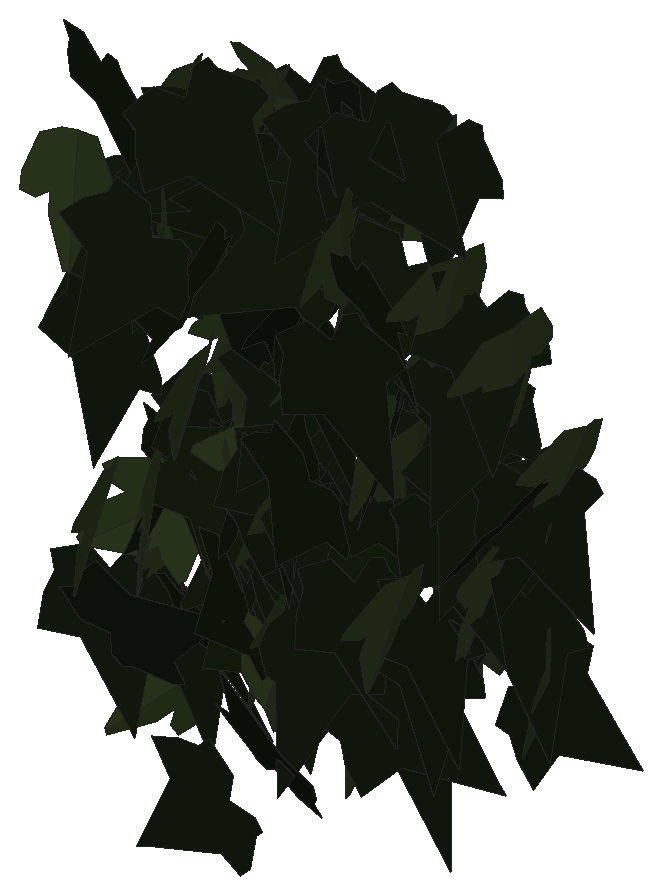
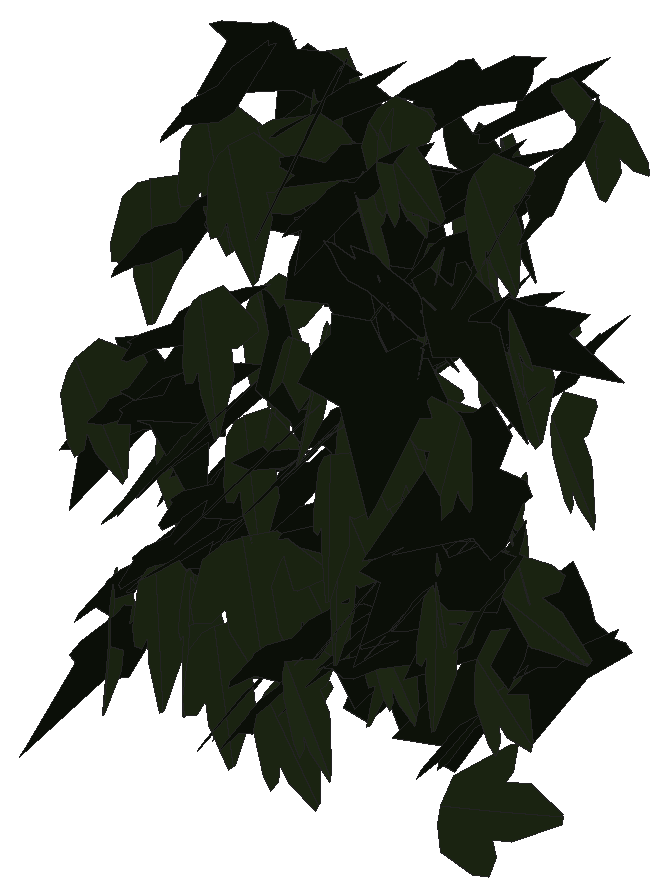
# SketchUp Ruby script. Lengths in inches.
U = 1.inch
M = Sketchup.active_model
def pt(a) = Geom::Point3d.new(a.map { |v| v * U })
def face(e, loops, mat)
  f = e.add_face(loops[0].map { |a| pt(a) })
  loops[1..].each { |l| e.add_face(l.map { |a| pt(a) }).erase! }
  f.material = f.back_material = mat if mat
  f
end
# faces: each face lists its corners as indices into pts; further lists are holes
def faces(e, pts, list, mat = nil) = list.each { |f| face(e, (f[0].is_a?(Array) ? f : [f]).map { |l| l.map { |i| pts[i] } }, mat) }
# xy, xz, yz: faces in a plane at the given z, y or x. An outline is a flat list of corners, or four numbers for a rectangle; further outlines are holes
def ring(l) = l.size == 4 ? [[l[0], l[1]], [l[2], l[1]], [l[2], l[3]], [l[0], l[3]]] : l.each_slice(2).to_a
def flat(e, list, mat, &to3) = list.each { |f| face(e, (f[0].is_a?(Array) ? f : [f]).map { |l| ring(l).map { |u, v| to3.(u, v) } }, mat) }
def xy(e, z, list, mat = nil) = flat(e, list, mat) { |x, y| [x, y, z] }
def xz(e, y, list, mat = nil) = flat(e, list, mat) { |x, z| [x, y, z] }
def yz(e, x, list, mat = nil) = flat(e, list, mat) { |y, z| [x, y, z] }
def lines(e, pts, list) = list.each { |a, b| e.add_line(pt(pts[a]), pt(pts[b])) }
# prism: a flat outline (further loops are holes) pulled along v
def prism(e, loops, v, mat = nil)
  f = face(e, loops, mat); d = Geom::Vector3d.new(v.map { |x| x * U })
  f.pushpull(f.normal.samedirection?(d) ? d.length : -d.length)
end
def box(e, o, s, mat = nil) = prism(e, [[o, [o[0] + s[0], o[1], o[2]], [o[0] + s[0], o[1] + s[1], o[2]], [o[0], o[1] + s[1], o[2]]]], [0, 0, s[2]], mat)
def at(x, y, z, deg = 0) = Geom::Transformation.translation(pt([x, y, z])) * Geom::Transformation.rotation(ORIGIN, Z_AXIS, deg.degrees)
def axes(o, x, y, z) = Geom::Transformation.new([*x, 0, *y, 0, *z, 0, *pt(o).to_a, 1])
def part(name) = M.definitions.add(name)
# library, detail: a bought-in or finely detailed component or shape, given as its bounding box
def library(name, o, s) = part(name).tap { |d| box(d.entities, o, s) }
def detail(e, o, s) = box(e.add_group.entities, o, s)
def put(e, d, t, mat = nil) = e.add_instance(d, t).tap { |i| i.material = mat if mat }
def group(e, t, mat = nil) = e.add_group.tap { |g| g.transformation = t; g.material = mat if mat }.entities
root = M.entities
M.materials.add("efeu1").color = [18, 25, 13]
M.materials.add("efeu2").color = [43, 57, 29]
c1 = part("ivyleaf_9")
p = [[1.54,2.16,1.25],[1.36,2.04,1.19],[-0.21,0.99,0.68],[-0.71,1.11,0.82],[-0.85,0.86,0.67],[-0.8,0.17,0.21],
  [-0.9,-0.01,0.1],[-0.67,-0.16,-0.02],[-0.08,-0.08,-0.05],[-0.03,-0.6,-0.4],[0.65,-0.88,-0.66],[0.83,-0.6,-0.49],
  [1.29,-0.42,-0.43],[1.8125,-0.07,-0.26],[1.21,0.44,0.15]]
faces(c1.entities,p,[[0,1,2,3,4,5,6,7,8,9,10,11,12,13,14]],"efeu1")
c2 = part("ivyleaf_10")
p = [[0,0.5,-0.03],[-0.0625,2.02,-0.43],[-0.19,2.01,-0.46],[-0.54,1.05,-0.29],[-0.52,0.625,-0.18],[-0.83,0.76,-0.28],
  [-1.16,0.64,-0.33],[-1.15,0.33,-0.24],[-0.77,-0.39,0.02],[-0.3,-0.51,0.16],[0.04,-0.48,0.23],[-0.02,2.01,-0.4375],
  [-0.06,2.01,-0.43],[0.04,-0.49,0.23],[0.67,-0.49,0.14],[1.38,0.36,-0.2],[1.375,0.51,-0.24],[0.81,0.65,-0.19],
  [0.62,0.59,-0.15],[0.6,1.09,-0.28],[0.5,1.23,-0.31]]
faces(c2.entities,p,[[0,1,2,3,4,5,6,7,8,9,10],[11,12,0,13,14,15,16,17,18,19,20]],"efeu2")
put(root,c1,axes([26.76,221.61,246.9],[-0.41542,-0.2389,0.14266],[-0.12264,-0.0729,-0.47921],[0.24977,-0.43314,0.00197]))
put(root,c1,axes([26.32,221.17,248.39],[0.2185,-0.41139,0.18169],[0.08102,-0.16269,-0.4658],[0.44237,0.233,-0.00443]))
put(root,c1,axes([26.38,222.13,245.81],[0.48589,0.05469,0.1045],[0.10564,-0.0048,-0.48869],[-0.05245,0.49698,-0.01621]))
put(root,c1,axes([26.5,221.06,243.3],[0.00566,-0.48604,-0.11717],[0.01799,0.1173,-0.48571],[0.49964,0.00128,0.01881]))
put(root,c2,axes([26.94,221.34,244.08],[0.30389,0.0047,-0.39703],[-0.39691,-0.00966,-0.30392],[-0.01053,0.49988,-0.00214]))
put(root,c2,axes([26.66,222.39,246.15],[-0.4394,0.22065,-0.09079],[0.05214,-0.09687,-0.48775],[-0.23284,-0.4381,0.06212]))
put(root,c1,axes([26.91,221.99,247.36],[-0.27595,0.40745,-0.08853],[0.02613,-0.08905,-0.49131],[-0.41613,-0.27578,0.02786]))
put(root,c2,axes([26.67,221.77,243.46],[0.13942,-0.41083,0.24856],[0.09036,-0.23175,-0.43373],[0.47159,0.16587,0.00963]))
put(root,c2,axes([26.85,221.89,242.1],[-0.059,-0.13773,0.47702],[-0.06244,-0.47451,-0.14472],[0.49257,-0.07664,0.03879]))
put(root,c2,axes([26.8125,221.3,246.59],[-0.06218,-0.48757,0.09172],[0.00454,-0.09299,-0.49126],[0.4961,-0.06026,0.01599]))
put(root,c2,axes([26.85,222.28,244.26],[0.06902,-0.46731,-0.16388],[0.01346,0.16717,-0.47103],[0.49503,0.06061,0.03565]))
put(root,c2,axes([26.84,221.64,248.19],[0.10371,-0.47786,0.10436],[0.02653,-0.10103,-0.48897],[0.48841,0.10696,0.0044]))
put(root,c2,axes([26.8,221.48,247.08],[0.3867,-0.30595,0.08279],[0.06813,-0.04731,-0.49307],[0.30955,0.39263,0.0051]))
put(root,c1,axes([26.91,221.35,244.12],[-0.0921,0.16964,-0.46124],[-0.21366,0.40877,0.19301],[0.44257,0.23265,-0.0028]))
put(root,c1,axes([26.72,220.8,246.05],[-0.00715,-0.47425,0.15823],[0.01944,-0.15839,-0.47385],[0.49957,-0.00062,0.0207]))
put(root,c1,axes([26.86,221.875,246.97],[-0.21036,-0.43707,0.12132],[-0.01661,-0.12622,-0.48352],[0.45329,-0.20746,0.03858]))
put(root,c1,axes([26.73,221.66,247.82],[0.29497,-0.39212,-0.09611],[-0.06557,0.07092,-0.49058],[0.39837,0.30202,-0.00959]))
put(root,c1,axes([26.69,221.87,244.23],[0.15079,-0.4088,0.24525],[0.10177,-0.22369,-0.43544],[0.46573,0.18123,0.01574]))
put(root,c1,axes([26.78,222.29,244.83],[0.00395,-0.30078,-0.39939],[0.0748,0.39527,-0.29693],[0.49436,-0.0574,0.04812]))
put(root,c2,axes([26.96,219.92,248.23],[0.48008,-0.07633,0.11703],[0.11589,-0.0164,-0.48611],[0.07805,0.49387,0.00195]))
put(root,c1,axes([26.92,221.67,242.94],[0.0946,-0.49092,-0.00722],[-0.00164,0.00703,-0.49995],[0.49097,0.09461,-0.00028]))
put(root,c1,axes([26.96,222.07,244.51],[0.02653,-0.49135,0.08874],[0.006,-0.08855,-0.49206],[0.49926,0.02718,0.00119]))
put(root,c2,axes([27.25,222.04,244.86],[0.27947,-0.33908,-0.23858],[-0.13923,0.19426,-0.43918],[0.39052,0.31191,0.01416]))
put(root,c2,axes([27,221.01,244.46],[0.25535,-0.31229,0.29542],[0.22377,-0.19683,-0.40148],[0.36705,0.33724,0.03924]))
put(root,c2,axes([27.27,222.16,245.86],[-0.04771,-0.47135,0.15986],[0.0196,-0.16225,-0.47254],[0.49733,-0.03883,0.03396]))
put(root,c1,axes([27.375,222.41,246.73],[0.08568,0.4926,0.00239],[-0.01319,0.00472,-0.4998],[-0.49243,0.08559,0.0138]))
put(root,c2,axes([27.34,221.78,247.31],[-0.32932,0.35214,0.13247],[-0.11034,0.07791,-0.48141],[-0.35968,-0.34631,0.0264]))
put(root,c2,axes([27.25,220.02,244.91],[0.20575,-0.43398,0.13902],[0.06484,-0.1231,-0.48025],[0.45107,0.21565,0.00562]))
put(root,c1,axes([26.9,220.63,243.06],[0.05921,-0.11064,0.484],[0.43949,-0.21506,-0.10293],[0.23095,0.43762,0.07179]))
put(root,c1,axes([27.22,221.45,247.64],[-0.01232,-0.49937,-0.02191],[0.00146,0.02188,-0.49952],[0.49985,-0.01237,0.00092]))
put(root,c1,axes([27.08,221.45,243.04],[0.36352,-0.33231,0.08613],[0.06164,-0.06021,-0.49252],[0.33771,0.3687,-0.00281]))
put(root,c1,axes([27.52,222.41,243.7],[-0.34521,-0.29662,0.20701],[-0.07847,-0.21792,-0.44312],[0.35309,-0.33842,0.1039]))
put(root,c1,axes([27.51,221.36,247.89],[-0.27384,-0.25936,0.32824],[-0.11521,-0.33039,-0.35717],[0.40217,-0.27125,0.12119]))
put(root,c1,axes([27.28,222.11,244.16],[0.05552,-0.46285,0.18081],[0.03828,-0.17741,-0.4659],[0.49543,0.06557,0.01574]))
put(root,c1,axes([27.67,222.37,247.56],[-0.49393,-0.02587,-0.07321],[0.07329,0.00028,-0.4946],[0.02563,-0.49933,0.00351]))
put(root,c2,axes([27.62,221.82,245.92],[0.01631,-0.49905,0.0262],[-0.00329,-0.02632,-0.4993],[0.49972,0.01611,-0.00414]))
put(root,c1,axes([27.47,221.65,244.52],[-0.15818,-0.46298,-0.10309],[0.04729,0.09274,-0.48904],[0.47196,-0.16447,0.01445]))
put(root,c1,axes([27.46,221.36,243.96],[-0.15151,0.41353,0.23673],[0.0715,-0.22587,0.44031],[0.4711,0.16727,0.0093]))
put(root,c2,axes([27.64,221.42,244.58],[-0.31331,0.3678,0.12867],[-0.08366,0.09776,-0.48316],[-0.38057,-0.32429,0.00028]))
put(root,c2,axes([27.93,221.67,248.41],[0.20225,0.00944,-0.45717],[-0.38418,0.27462,-0.16429],[0.248,0.41772,0.11834]))
put(root,c2,axes([27.79,221.78,244.6875],[-0.31598,-0.31948,0.21929],[-0.035,-0.25827,-0.4267],[0.38592,-0.285,0.14086]))
put(root,c2,axes([27.72,220.23,247.58],[0.2344,-0.41132,-0.16084],[-0.02058,0.17172,-0.46914],[0.44117,0.22655,0.06358]))
put(root,c2,axes([27.75,222.66,245.43],[0.08858,-0.4574,-0.18148],[-0.00223,0.18402,-0.4649],[0.49209,0.08317,0.03056]))
put(root,c2,axes([27.88,222.39,244.625],[0.10187,-0.42934,-0.23513],[-0.03606,0.23293,-0.44096],[0.48818,0.1068,0.01649]))
put(root,c2,axes([27.8,221.75,248.39],[0.15506,-0.44108,0.1772],[0.06878,-0.16361,-0.46744],[0.47035,0.16934,0.00994]))
put(root,c1,axes([27.7,222.24,244.18],[0.21035,-0.45326,-0.01771],[-0.00686,0.01634,-0.49969],[0.45355,0.21046,0.00066]))
put(root,c2,axes([27.95,221.9375,247.77],[0.27346,-0.41824,0.01706],[0.00605,-0.01643,-0.49969],[0.41855,0.2735,-0.00393]))
put(root,c1,axes([27.71,220.67,248.73],[0.1066,-0.36964,-0.31938],[0.07193,0.3352,-0.36396],[0.48318,0.03165,0.12464]))
put(root,c1,axes([28.01,219.71,247.85],[-0.20848,-0.39819,0.21904],[-0.02795,-0.2293,-0.44344],[0.4536,-0.19714,0.07336]))
put(root,c1,axes([28.26,221.51,247.55],[-0.12426,-0.25443,-0.4121],[-0.04931,-0.41659,0.27207],[-0.4818,0.10825,0.07844]))
put(root,c1,axes([27.96,221.21,243.45],[-0.11712,-0.1772,0.45264],[0.00905,-0.46631,-0.1802],[0.486,-0.03402,0.11244]))
put(root,c1,axes([27.85,221.9,243.69],[0.2715,-0.35175,-0.22926],[-0.03182,0.25499,-0.42892],[0.41866,0.24749,0.11607]))
put(root,c1,axes([27.88,222.23,248.23],[0.12201,-0.44989,-0.18087],[-0.00995,0.18415,-0.46475],[0.48478,0.11701,0.03599]))
put(root,c2,axes([28.08,221.53,243.27],[0.19335,-0.44178,0.13209],[0.03945,-0.12686,-0.48203],[0.45941,0.19682,-0.0142]))
put(root,c2,axes([28.1,221.92,245.47],[0.11748,-0.44415,0.19731],[0.0812,-0.1822,-0.45849],[0.47917,0.13977,0.02931]))
put(root,c1,axes([28.27,221.01,246.86],[0.27788,0.25343,-0.32948],[-0.25333,-0.21097,-0.37592],[-0.32956,0.37585,0.01115]))
put(root,c1,axes([28.4375,219.8,247.42],[-0.25722,0.40946,0.12721],[-0.078,0.10118,-0.4834],[-0.42161,-0.26852,0.01182]))
put(root,c2,axes([28.33,221.02,242.84],[0.06146,0.21093,-0.44914],[-0.04464,0.45309,0.20668],[0.4942,0.01469,0.07452]))
put(root,c1,axes([28.13,222.76,243.78],[-0.05439,-0.49695,-0.00913],[0.03015,0.00587,-0.49906],[0.49612,-0.05484,0.02933]))
put(root,c2,axes([28.28,222.49,243.14],[0.17616,-0.45619,0.10418],[0.03133,-0.09957,-0.48898],[0.46689,0.17881,-0.0065]))
put(root,c1,axes([28.22,221.67,245.54],[-0.1988,-0.38449,0.25029],[0.04144,-0.28671,-0.40753],[0.45691,-0.14128,0.14586]))
put(root,c1,axes([28.2,221.47,243.36],[-0.14028,-0.42065,-0.23103],[0.10856,0.20664,-0.44217],[0.46748,-0.17422,0.03336]))
put(root,c1,axes([28.24,222.06,245.52],[-0.01795,-0.45535,0.20576],[0.06734,-0.20622,-0.45049],[0.49512,0.01154,0.06873]))
put(root,c2,axes([28.46,219.85,246.67],[0.1399,-0.47991,0.01066],[0.00168,-0.01061,-0.49988],[0.48003,0.13991,-0.00136]))
put(root,c2,axes([28.55,222.08,244],[-0.01307,-0.46776,0.17615],[-0.00512,-0.17608,-0.46794],[0.4998,-0.01403,-0.00019]))
put(root,c2,axes([28.5625,220.89,244.91],[0.03567,-0.45238,-0.20996],[0.00924,0.21106,-0.45317],[0.49864,0.02845,0.02342]))
put(root,c2,axes([28.57,221.74,246.0625],[0.14008,-0.36365,-0.31327],[0.01563,0.32962,-0.37565],[0.47972,0.09545,0.10371]))
put(root,c1,axes([28.34,220.9,244.76],[0.35963,-0.31579,-0.14471],[-0.03846,0.17081,-0.46834],[0.34523,0.348,0.09857]))
put(root,c1,axes([28.73,221.15,246.9],[-0.03242,0.47828,-0.14213],[0.00695,-0.14198,-0.47937],[-0.4989,-0.03306,0.00255]))
put(root,c1,axes([28.41,221.16,245.26],[-0.24565,-0.05603,-0.43188],[0.43414,0.00767,-0.24793],[0.03441,-0.49679,0.04488]))
put(root,c1,axes([28.58,220.8,242.19],[0.38005,-0.28491,0.15616],[-0.11947,0.10093,0.47491],[-0.30214,-0.39829,0.00864]))
put(root,c1,axes([28.75,221.16,247.44],[-0.32583,-0.24294,0.29123],[-0.17372,-0.2457,-0.39932],[0.33713,-0.3614,0.0757]))
put(root,c1,axes([28.45,221.53,246.12],[0.206,-0.45146,0.0612],[0.0244,-0.05613,-0.49624],[0.45494,0.20744,-0.00109]))
put(root,c1,axes([28.67,221.59,247.87],[-0.27168,-0.39731,-0.13541],[0.06122,0.12206,-0.48099],[0.41526,-0.27794,-0.01767]))
put(root,c1,axes([28.6,221.09,245.23],[-0.0633,-0.48089,-0.12138],[0.0373,0.11741,-0.48459],[0.49457,-0.0704,0.02101]))
put(root,c2,axes([28.84,222.53,244.16],[-0.28212,-0.40697,0.06918],[-0.0191,-0.07084,-0.49459],[0.41237,-0.2817,0.02443]))
put(root,c1,axes([28.78,221.43,248.52],[0.28392,-0.12684,-0.39153],[-0.30129,0.25999,-0.30271],[0.28038,0.40782,0.0712]))
put(root,c2,axes([28.84,222.07,242.44],[0.07398,-0.47027,0.15287],[0.01271,-0.15272,-0.47594],[0.49433,0.0743,-0.01064]))
put(root,c1,axes([28.61,222.39,242.96],[0.11861,-0.48488,0.02865],[0.00477,-0.02833,-0.49917],[0.4857,0.11869,-0.0021]))
put(root,c1,axes([28.82,222.21,244.17],[-0.23062,-0.43573,-0.08341],[0.03282,0.07699,-0.49295],[0.44242,-0.23284,-0.00691]))
put(root,c1,axes([28.66,222.375,245.36],[0.29685,-0.34539,-0.20636],[-0.04125,0.22897,-0.44257],[0.40023,0.27978,0.10744]))
put(root,c1,axes([28.87,221.53,248.31],[-0.20931,-0.4004,0.21418],[-0.01544,-0.22943,-0.44399],[0.45382,-0.19247,0.08367]))
put(root,c1,axes([28.92,221.15,243.4375],[-0.42209,-0.16759,-0.20917],[0.20331,0.05407,-0.45359],[0.17465,-0.46796,0.02251]))
put(root,c2,axes([28.76,221.5,247.89],[-0.24669,-0.12477,-0.41662],[0.38525,0.15957,-0.2759],[0.20181,-0.45713,0.01741]))
put(root,c2,axes([29.0625,222.39,247.99],[-0.00137,-0.49978,0.01489],[0.00024,-0.01489,-0.49978],[0.5,-0.00136,0.00028]))
put(root,c2,axes([29.09,222.16,245.14],[0.03413,-0.49381,-0.07059],[-0.00782,0.07022,-0.49498],[0.49877,0.03489,-0.00293]))
put(root,c1,axes([28.87,221.74,244.875],[0.28571,-0.34818,-0.21712],[-0.05752,0.22796,-0.44127],[0.40627,0.27713,0.09021]))
put(root,c2,axes([29.28,221.37,245.51],[0.10959,-0.40545,-0.27129],[0.0494,0.28584,-0.40725],[0.48534,0.06246,0.1027]))
put(root,c2,axes([29.33,222.47,246.41],[0.05469,-0.49319,-0.06142],[0.00069,0.06186,-0.49616],[0.497,0.05419,0.00744]))
put(root,c1,axes([29.13,220.6,245.37],[-0.08171,-0.34922,0.34838],[0.08904,-0.35777,-0.33775],[0.48518,0.00684,0.12066]))
put(root,c1,axes([29.25,222.45,244.82],[-0.1634,-0.4689,0.05855],[-0.0005,-0.06177,-0.49617],[0.47254,-0.16221,0.01972]))
put(root,c1,axes([29.5,221.07,245.27],[0.04299,0.11665,0.4843],[-0.01192,0.4862,-0.11605],[-0.49801,-0.00157,0.04459]))
put(root,c2,axes([29.43,220.62,248.03],[0.10949,-0.45826,-0.16737],[0.03188,0.17788,-0.4662],[0.48682,0.09141,0.06817]))
put(root,c2,axes([29.48,222.1,242.84],[-0.06773,-0.49524,-0.01206],[0.00097,0.01204,-0.49985],[0.49539,-0.06774,-0.00066]))
put(root,c1,axes([29.3,221.85,242.51],[0.17674,-0.46771,-0.00385],[-0.00054,0.00391,-0.49998],[0.46772,0.17674,0.00088]))
put(root,c1,axes([29.52,221.48,247.28],[-0.24767,-0.43313,0.03254],[-0.01204,-0.0306,-0.49892],[0.43419,-0.24791,0.00473]))
put(root,c1,axes([29.26,221.35,248.72],[-0.00516,-0.28895,-0.40802],[0.31651,0.31398,-0.22636],[0.38704,-0.26061,0.17967]))
put(root,c1,axes([29.44,222.69,245.19],[-0.04556,-0.43913,0.23471],[0.03098,-0.23773,-0.43878],[0.49696,-0.02544,0.04887]))
put(root,c1,axes([29.44,220.89,244.27],[0.07772,-0.47492,-0.13567],[0.00165,0.13759,-0.48069],[0.49392,0.07428,0.02296]))
put(root,c2,axes([29.77,222.09,243.28],[0.08765,-0.39063,-0.29955],[-0.05276,0.29505,-0.4002],[0.48942,0.10176,0.0105]))
put(root,c2,axes([29.79,222.5625,243.55],[0.03387,-0.48136,-0.13096],[-0.01417,0.13028,-0.48252],[0.49865,0.0364,-0.00482]))
put(root,c1,axes([29.63,221.9375,248.49],[-0.01099,-0.49655,0.05759],[0.0074,-0.05776,-0.4966],[0.49982,-0.01006,0.00862]))
put(root,c1,axes([29.68,222.42,243.93],[-0.12776,-0.45063,0.17497],[0.06325,-0.195,-0.45604],[0.47925,-0.09439,0.10683]))
put(root,c1,axes([29.52,220.85,247.51],[0.26113,-0.38801,0.1768],[0.09589,-0.14858,-0.46769],[0.41547,0.27816,-0.00319]))
put(root,c1,axes([29.72,222.47,244.14],[-0.07294,-0.48716,0.08575],[-0.01556,-0.08438,-0.49258],[0.49441,-0.07453,-0.00285]))
put(root,c2,axes([30.12,221.4,247.49],[-0.05341,-0.49694,0.01411],[-0.00126,-0.01405,-0.4998],[0.49714,-0.05343,0.00025]))
put(root,c1,axes([30.02,222.07,246.01],[-0.19488,-0.44531,0.11714],[0.01191,-0.13204,-0.4821],[0.4603,-0.18512,0.06208]))
put(root,c1,axes([29.91,221.52,244.875],[0.19538,-0.43138,-0.16044],[-0.03489,0.15992,-0.47245],[0.45892,0.19581,0.03239]))
put(root,c1,axes([29.96,222.49,244.64],[-0.01302,-0.42906,0.25639],[0.08193,-0.25484,-0.42231],[0.49307,0.03102,0.07694]))
put(root,c1,axes([30.14,222.03,245.22],[-0.20546,-0.45148,0.06289],[-0.01707,-0.06132,-0.49593],[0.45552,-0.20593,0.00978]))
put(root,c1,axes([30,220.67,243.4375],[0.06994,-0.19559,-0.45481],[0.01813,0.46003,-0.19505],[0.49475,0.0108,0.07144]))
put(root,c1,axes([30.04,219.83,247.42],[-0.19864,-0.13614,-0.43819],[0.35678,0.25442,-0.24079],[0.28853,-0.40833,-0.00393]))
put(root,c1,axes([30.15,221.87,246.89],[-0.00925,-0.49817,-0.0417],[0.00932,0.04153,-0.49819],[0.49983,-0.01,0.00851]))
put(root,c1,axes([30.3,217.95,243.69],[-0.24256,-0.23166,0.37081],[-0.01177,-0.42044,-0.27036],[0.43706,-0.13989,0.19851]))
put(root,c1,axes([30.15,222.43,243.7],[0.07989,-0.49304,-0.02298],[0.01091,0.02504,-0.49925],[0.49346,0.07927,0.01476]))
put(root,c1,axes([30.14,221.03,244.23],[0.1347,-0.48118,-0.01805],[-0.00525,0.01728,-0.49967],[0.48149,0.1348,-0.0004]))
put(root,c1,axes([30.62,221.44,245.07],[-0.14411,0.47827,-0.02215],[-0.00918,-0.02588,-0.49925],[-0.47869,-0.14349,0.01624]))
put(root,c2,axes([30.37,221.67,244.39],[0.1634,-0.38842,0.26912],[0.10858,-0.24628,-0.42138],[0.4599,0.19615,0.00387]))
put(root,c2,axes([30.49,222.27,243.12],[0.13547,-0.35728,-0.32249],[-0.04691,0.32363,-0.37824],[0.47901,0.13274,0.05417]))
put(root,c1,axes([30.27,220.92,244.03],[0.05753,-0.49225,0.06618],[-0.00278,-0.06694,-0.49549],[0.49667,0.05664,-0.01044]))
put(root,c1,axes([30.34,222.38,242.93],[0.21194,-0.18272,-0.41436],[-0.17068,0.39153,-0.25995],[0.41947,0.25163,0.10359]))
put(root,c2,axes([30.5625,221.7,246.81],[-0.09112,-0.485,-0.08043],[0.01533,0.07896,-0.49349],[0.49139,-0.09239,0.00048]))
put(root,c2,axes([30.59,220.04,244.97],[0.05047,-0.49206,0.07301],[-0.00134,-0.07352,-0.49456],[0.49744,0.04972,-0.00874]))
put(root,c2,axes([30.6,222.56,245.4],[0.04389,-0.4841,0.11712],[-0.00461,-0.11797,-0.48586],[0.49805,0.04157,-0.01482]))
put(root,c1,axes([30.4,222.18,245.1],[0.09434,-0.41744,-0.25855],[-0.0276,0.25835,-0.42719],[0.49024,0.09487,0.0257]))
